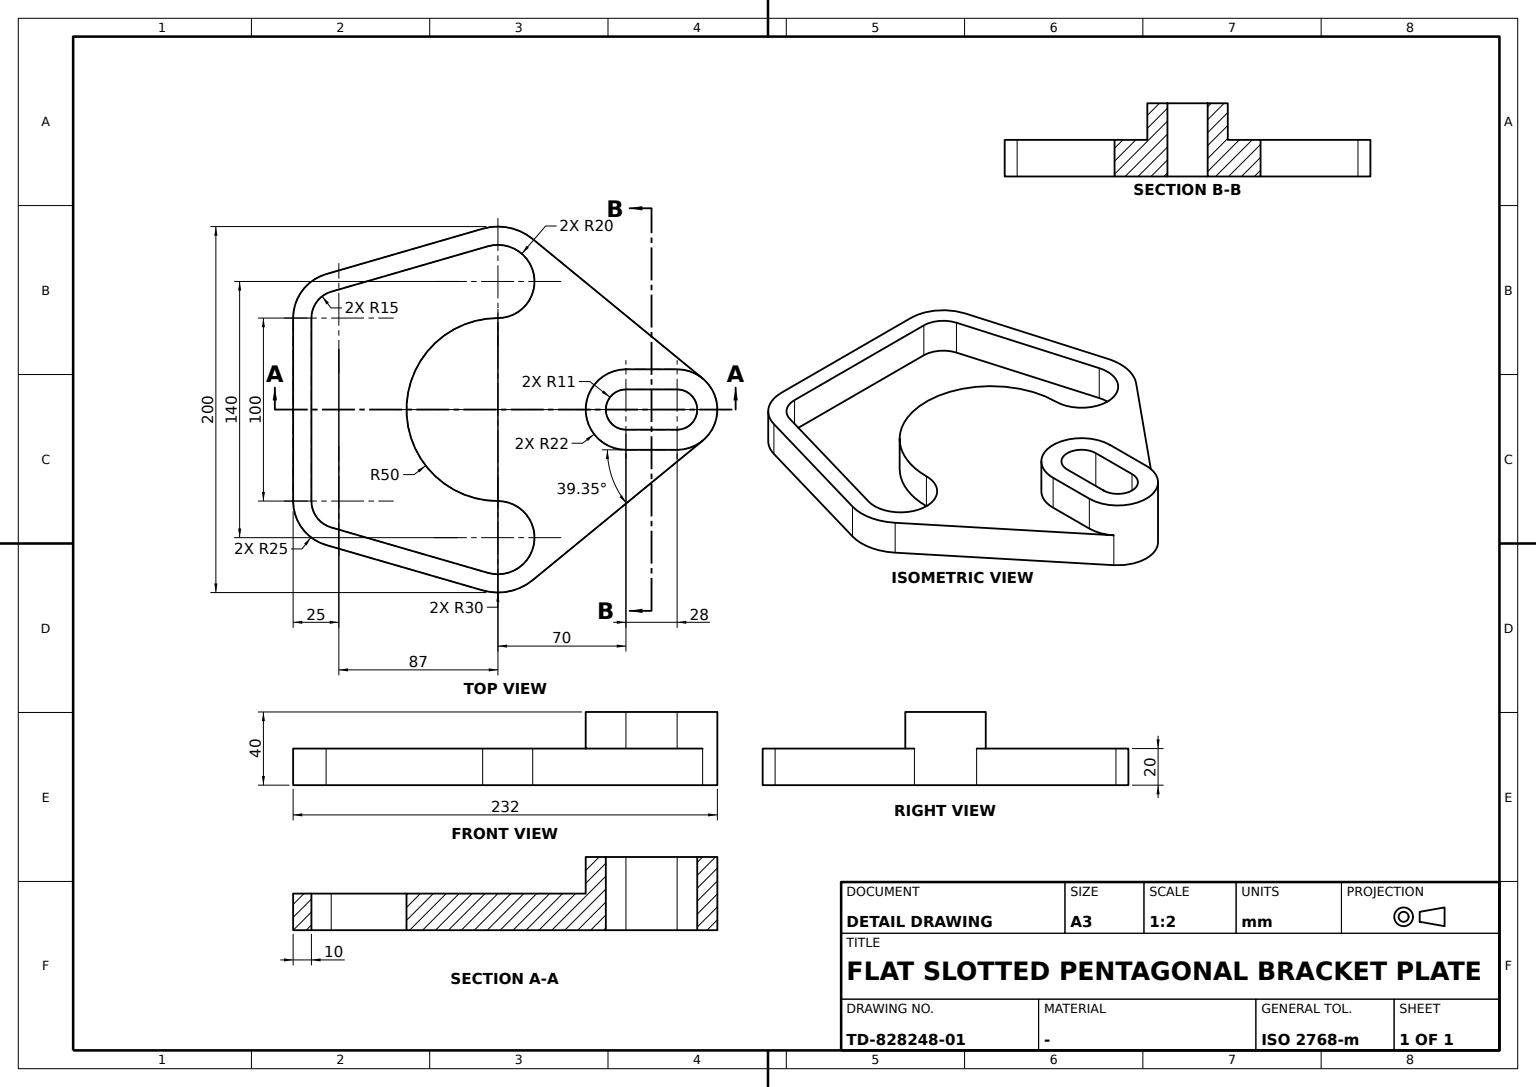
ISO-10303-21;
HEADER;
FILE_DESCRIPTION((''),'2;1');
FILE_NAME('','',(''),(''),'','','');
FILE_SCHEMA(('AUTOMOTIVE_DESIGN'));
ENDSEC;
DATA;
#1=APPLICATION_CONTEXT('');
#2=PRODUCT_CONTEXT('',#1,'mechanical');
#3=PRODUCT('','','',(#2));
#4=PRODUCT_DEFINITION_FORMATION('','',#3);
#5=PRODUCT_DEFINITION_CONTEXT('',#1,'design');
#6=PRODUCT_DEFINITION('','',#4,#5);
#7=PRODUCT_DEFINITION_SHAPE('','',#6);
#8=(LENGTH_UNIT()NAMED_UNIT(*)SI_UNIT(.MILLI.,.METRE.));
#9=(NAMED_UNIT(*)PLANE_ANGLE_UNIT()SI_UNIT($,.RADIAN.));
#10=(NAMED_UNIT(*)SI_UNIT($,.STERADIAN.)SOLID_ANGLE_UNIT());
#11=UNCERTAINTY_MEASURE_WITH_UNIT(LENGTH_MEASURE(0.005),#8,'distance_accuracy_value','');
#12=(GEOMETRIC_REPRESENTATION_CONTEXT(3)GLOBAL_UNCERTAINTY_ASSIGNED_CONTEXT((#11))GLOBAL_UNIT_ASSIGNED_CONTEXT((#8,#9,#10))REPRESENTATION_CONTEXT('',''));
#13=CARTESIAN_POINT('',(64.407517,-91.174142,0.));
#14=VERTEX_POINT('',#13);
#15=CARTESIAN_POINT('',(64.407517,-91.174142,-20.));
#16=VERTEX_POINT('',#15);
#17=CARTESIAN_POINT('',(64.407517,-91.174142,-10.));
#18=DIRECTION('',(0.,0.,1.));
#19=VECTOR('',#18,1000.);
#20=LINE('',#17,#19);
#21=EDGE_CURVE('',#14,#16,#20,.F.);
#22=ORIENTED_EDGE('',*,*,#21,.F.);
#23=CARTESIAN_POINT('',(89.210022,-5.565522,0.));
#24=VERTEX_POINT('',#23);
#25=DIRECTION('',(0.27827612,0.96050112,0.));
#26=VECTOR('',#25,1000.);
#27=LINE('',#13,#26);
#28=EDGE_CURVE('',#14,#24,#27,.T.);
#29=ORIENTED_EDGE('',*,*,#28,.T.);
#30=CARTESIAN_POINT('',(89.210022,-5.565522,-20.));
#31=VERTEX_POINT('',#30);
#32=CARTESIAN_POINT('',(89.210022,-5.565522,-10.));
#33=LINE('',#32,#19);
#34=EDGE_CURVE('',#24,#31,#33,.F.);
#35=ORIENTED_EDGE('',*,*,#34,.T.);
#36=LINE('',#15,#26);
#37=EDGE_CURVE('',#16,#31,#36,.T.);
#38=ORIENTED_EDGE('',*,*,#37,.F.);
#39=EDGE_LOOP('',(#22,#29,#35,#38));
#40=FACE_BOUND('',#39,.T.);
#41=DIRECTION('',(-0.96050112,0.27827612,0.));
#42=AXIS2_PLACEMENT_3D('',#13,#41,#25);
#43=PLANE('',#42);
#44=ADVANCED_FACE('',(#40),#43,.T.);
#45=CARTESIAN_POINT('',(-11.,70.,20.));
#46=VERTEX_POINT('',#45);
#47=CARTESIAN_POINT('',(-11.,70.,-20.));
#48=VERTEX_POINT('',#47);
#49=CARTESIAN_POINT('',(-11.,70.,10.));
#50=LINE('',#49,#19);
#51=EDGE_CURVE('',#46,#48,#50,.F.);
#52=ORIENTED_EDGE('',*,*,#51,.F.);
#53=CARTESIAN_POINT('',(11.,70.,20.));
#54=VERTEX_POINT('',#53);
#55=CARTESIAN_POINT('',(0.,70.,20.));
#56=DIRECTION('',(1.,0.,0.));
#57=AXIS2_PLACEMENT_3D('',#55,#18,#56);
#58=CIRCLE('',#57,11.);
#59=EDGE_CURVE('',#46,#54,#58,.T.);
#60=ORIENTED_EDGE('',*,*,#59,.T.);
#61=CARTESIAN_POINT('',(11.,70.,-20.));
#62=VERTEX_POINT('',#61);
#63=CARTESIAN_POINT('',(11.,70.,10.));
#64=LINE('',#63,#19);
#65=EDGE_CURVE('',#54,#62,#64,.F.);
#66=ORIENTED_EDGE('',*,*,#65,.T.);
#67=CARTESIAN_POINT('',(0.,70.,-20.));
#68=AXIS2_PLACEMENT_3D('',#67,#18,#56);
#69=CIRCLE('',#68,11.);
#70=EDGE_CURVE('',#48,#62,#69,.T.);
#71=ORIENTED_EDGE('',*,*,#70,.F.);
#72=EDGE_LOOP('',(#52,#60,#66,#71));
#73=FACE_BOUND('',#72,.T.);
#74=CARTESIAN_POINT('',(0.,70.,10.));
#75=AXIS2_PLACEMENT_3D('',#74,#18,#56);
#76=CYLINDRICAL_SURFACE('',#75,11.);
#77=ADVANCED_FACE('',(#73),#76,.F.);
#78=CARTESIAN_POINT('',(98.815034,-8.348284,-20.));
#79=VERTEX_POINT('',#78);
#80=CARTESIAN_POINT('',(93.199784,19.020254,-20.));
#81=VERTEX_POINT('',#80);
#82=CARTESIAN_POINT('',(70.,0.,-20.));
#83=AXIS2_PLACEMENT_3D('',#82,#18,#56);
#84=CIRCLE('',#83,30.);
#85=EDGE_CURVE('',#79,#81,#84,.T.);
#86=ORIENTED_EDGE('',*,*,#85,.T.);
#87=CARTESIAN_POINT('',(93.199784,19.020254,0.));
#88=VERTEX_POINT('',#87);
#89=CARTESIAN_POINT('',(93.199784,19.020254,-10.));
#90=LINE('',#89,#19);
#91=EDGE_CURVE('',#88,#81,#90,.F.);
#92=ORIENTED_EDGE('',*,*,#91,.F.);
#93=CARTESIAN_POINT('',(98.815034,-8.348284,0.));
#94=VERTEX_POINT('',#93);
#95=CARTESIAN_POINT('',(70.,0.,0.));
#96=AXIS2_PLACEMENT_3D('',#95,#18,#56);
#97=CIRCLE('',#96,30.);
#98=EDGE_CURVE('',#94,#88,#97,.T.);
#99=ORIENTED_EDGE('',*,*,#98,.F.);
#100=CARTESIAN_POINT('',(98.815034,-8.348284,-10.));
#101=LINE('',#100,#19);
#102=EDGE_CURVE('',#94,#79,#101,.F.);
#103=ORIENTED_EDGE('',*,*,#102,.T.);
#104=EDGE_LOOP('',(#86,#92,#99,#103));
#105=FACE_BOUND('',#104,.T.);
#106=CARTESIAN_POINT('',(70.,0.,-10.));
#107=AXIS2_PLACEMENT_3D('',#106,#18,#56);
#108=CYLINDRICAL_SURFACE('',#107,30.);
#109=ADVANCED_FACE('',(#105),#108,.T.);
#110=CARTESIAN_POINT('',(22.,70.,0.));
#111=VERTEX_POINT('',#110);
#112=CARTESIAN_POINT('',(22.,70.,20.));
#113=VERTEX_POINT('',#112);
#114=CARTESIAN_POINT('',(22.,70.,10.));
#115=LINE('',#114,#19);
#116=EDGE_CURVE('',#111,#113,#115,.T.);
#117=ORIENTED_EDGE('',*,*,#116,.T.);
#118=CARTESIAN_POINT('',(-22.,70.,20.));
#119=VERTEX_POINT('',#118);
#120=CIRCLE('',#57,22.);
#121=EDGE_CURVE('',#119,#113,#120,.T.);
#122=ORIENTED_EDGE('',*,*,#121,.F.);
#123=CARTESIAN_POINT('',(-22.,70.,0.));
#124=VERTEX_POINT('',#123);
#125=CARTESIAN_POINT('',(-22.,70.,10.));
#126=LINE('',#125,#19);
#127=EDGE_CURVE('',#124,#119,#126,.T.);
#128=ORIENTED_EDGE('',*,*,#127,.F.);
#129=CARTESIAN_POINT('',(0.,70.,0.));
#130=AXIS2_PLACEMENT_3D('',#129,#18,#56);
#131=CIRCLE('',#130,22.);
#132=EDGE_CURVE('',#124,#111,#131,.T.);
#133=ORIENTED_EDGE('',*,*,#132,.T.);
#134=EDGE_LOOP('',(#117,#122,#128,#133));
#135=FACE_BOUND('',#134,.T.);
#136=CYLINDRICAL_SURFACE('',#75,22.);
#137=ADVANCED_FACE('',(#135),#136,.T.);
#138=CARTESIAN_POINT('',(-64.407517,-91.174142,0.));
#139=VERTEX_POINT('',#138);
#140=CARTESIAN_POINT('',(-89.210022,-5.565522,0.));
#141=VERTEX_POINT('',#140);
#142=DIRECTION('',(-0.27827612,0.96050112,0.));
#143=VECTOR('',#142,1000.);
#144=LINE('',#138,#143);
#145=EDGE_CURVE('',#139,#141,#144,.T.);
#146=ORIENTED_EDGE('',*,*,#145,.F.);
#147=CARTESIAN_POINT('',(-64.407517,-91.174142,-20.));
#148=VERTEX_POINT('',#147);
#149=CARTESIAN_POINT('',(-64.407517,-91.174142,-10.));
#150=LINE('',#149,#19);
#151=EDGE_CURVE('',#139,#148,#150,.F.);
#152=ORIENTED_EDGE('',*,*,#151,.T.);
#153=CARTESIAN_POINT('',(-89.210022,-5.565522,-20.));
#154=VERTEX_POINT('',#153);
#155=LINE('',#147,#143);
#156=EDGE_CURVE('',#148,#154,#155,.T.);
#157=ORIENTED_EDGE('',*,*,#156,.T.);
#158=CARTESIAN_POINT('',(-89.210022,-5.565522,-10.));
#159=LINE('',#158,#19);
#160=EDGE_CURVE('',#141,#154,#159,.F.);
#161=ORIENTED_EDGE('',*,*,#160,.F.);
#162=EDGE_LOOP('',(#146,#152,#157,#161));
#163=FACE_BOUND('',#162,.T.);
#164=DIRECTION('',(-0.96050112,-0.27827612,0.));
#165=AXIS2_PLACEMENT_3D('',#138,#164,#142);
#166=PLANE('',#165);
#167=ADVANCED_FACE('',(#163),#166,.F.);
#168=CARTESIAN_POINT('',(11.,98.,20.));
#169=VERTEX_POINT('',#168);
#170=CARTESIAN_POINT('',(-11.,98.,20.));
#171=VERTEX_POINT('',#170);
#172=CARTESIAN_POINT('',(0.,98.,20.));
#173=AXIS2_PLACEMENT_3D('',#172,#18,#56);
#174=CIRCLE('',#173,11.);
#175=EDGE_CURVE('',#169,#171,#174,.T.);
#176=ORIENTED_EDGE('',*,*,#175,.T.);
#177=CARTESIAN_POINT('',(-11.,98.,-20.));
#178=VERTEX_POINT('',#177);
#179=CARTESIAN_POINT('',(-11.,98.,10.));
#180=LINE('',#179,#19);
#181=EDGE_CURVE('',#171,#178,#180,.F.);
#182=ORIENTED_EDGE('',*,*,#181,.T.);
#183=CARTESIAN_POINT('',(11.,98.,-20.));
#184=VERTEX_POINT('',#183);
#185=CARTESIAN_POINT('',(0.,98.,-20.));
#186=AXIS2_PLACEMENT_3D('',#185,#18,#56);
#187=CIRCLE('',#186,11.);
#188=EDGE_CURVE('',#184,#178,#187,.T.);
#189=ORIENTED_EDGE('',*,*,#188,.F.);
#190=CARTESIAN_POINT('',(11.,98.,10.));
#191=LINE('',#190,#19);
#192=EDGE_CURVE('',#169,#184,#191,.F.);
#193=ORIENTED_EDGE('',*,*,#192,.F.);
#194=EDGE_LOOP('',(#176,#182,#189,#193));
#195=FACE_BOUND('',#194,.T.);
#196=CARTESIAN_POINT('',(0.,98.,10.));
#197=AXIS2_PLACEMENT_3D('',#196,#18,#56);
#198=CYLINDRICAL_SURFACE('',#197,11.);
#199=ADVANCED_FACE('',(#195),#198,.F.);
#200=ORIENTED_EDGE('',*,*,#59,.F.);
#201=CARTESIAN_POINT('',(-11.,0.,20.));
#202=DIRECTION('',(0.,1.,0.));
#203=VECTOR('',#202,1000.);
#204=LINE('',#201,#203);
#205=EDGE_CURVE('',#46,#171,#204,.T.);
#206=ORIENTED_EDGE('',*,*,#205,.T.);
#207=ORIENTED_EDGE('',*,*,#175,.F.);
#208=CARTESIAN_POINT('',(11.,0.,20.));
#209=DIRECTION('',(0.,-1.,0.));
#210=VECTOR('',#209,1000.);
#211=LINE('',#208,#210);
#212=EDGE_CURVE('',#169,#54,#211,.T.);
#213=ORIENTED_EDGE('',*,*,#212,.T.);
#214=EDGE_LOOP('',(#200,#206,#207,#213));
#215=FACE_BOUND('',#214,.T.);
#216=CARTESIAN_POINT('',(22.,98.,20.));
#217=VERTEX_POINT('',#216);
#218=CARTESIAN_POINT('',(22.,0.,20.));
#219=LINE('',#218,#210);
#220=EDGE_CURVE('',#217,#113,#219,.T.);
#221=ORIENTED_EDGE('',*,*,#220,.F.);
#222=CARTESIAN_POINT('',(-22.,98.,20.));
#223=VERTEX_POINT('',#222);
#224=CIRCLE('',#173,22.);
#225=EDGE_CURVE('',#217,#223,#224,.T.);
#226=ORIENTED_EDGE('',*,*,#225,.T.);
#227=CARTESIAN_POINT('',(-22.,0.,20.));
#228=LINE('',#227,#203);
#229=EDGE_CURVE('',#119,#223,#228,.T.);
#230=ORIENTED_EDGE('',*,*,#229,.F.);
#231=ORIENTED_EDGE('',*,*,#121,.T.);
#232=EDGE_LOOP('',(#221,#226,#230,#231));
#233=FACE_BOUND('',#232,.T.);
#234=CARTESIAN_POINT('',(0.,0.,20.));
#235=AXIS2_PLACEMENT_3D('',#234,#18,#56);
#236=PLANE('',#235);
#237=ADVANCED_FACE('',(#215,#233),#236,.T.);
#238=CARTESIAN_POINT('',(-93.199784,19.020254,0.));
#239=VERTEX_POINT('',#238);
#240=CARTESIAN_POINT('',(-98.815034,-8.348284,0.));
#241=VERTEX_POINT('',#240);
#242=CARTESIAN_POINT('',(-70.,0.,0.));
#243=AXIS2_PLACEMENT_3D('',#242,#18,#56);
#244=CIRCLE('',#243,30.);
#245=EDGE_CURVE('',#239,#241,#244,.T.);
#246=ORIENTED_EDGE('',*,*,#245,.F.);
#247=CARTESIAN_POINT('',(-93.199784,19.020254,-20.));
#248=VERTEX_POINT('',#247);
#249=CARTESIAN_POINT('',(-93.199784,19.020254,-10.));
#250=LINE('',#249,#19);
#251=EDGE_CURVE('',#239,#248,#250,.F.);
#252=ORIENTED_EDGE('',*,*,#251,.T.);
#253=CARTESIAN_POINT('',(-98.815034,-8.348284,-20.));
#254=VERTEX_POINT('',#253);
#255=CARTESIAN_POINT('',(-70.,0.,-20.));
#256=AXIS2_PLACEMENT_3D('',#255,#18,#56);
#257=CIRCLE('',#256,30.);
#258=EDGE_CURVE('',#248,#254,#257,.T.);
#259=ORIENTED_EDGE('',*,*,#258,.T.);
#260=CARTESIAN_POINT('',(-98.815034,-8.348284,-10.));
#261=LINE('',#260,#19);
#262=EDGE_CURVE('',#241,#254,#261,.F.);
#263=ORIENTED_EDGE('',*,*,#262,.F.);
#264=EDGE_LOOP('',(#246,#252,#259,#263));
#265=FACE_BOUND('',#264,.T.);
#266=CARTESIAN_POINT('',(-70.,0.,-10.));
#267=AXIS2_PLACEMENT_3D('',#266,#18,#56);
#268=CYLINDRICAL_SURFACE('',#267,30.);
#269=ADVANCED_FACE('',(#265),#268,.T.);
#270=CARTESIAN_POINT('',(50.,0.,0.));
#271=VERTEX_POINT('',#270);
#272=CARTESIAN_POINT('',(50.,0.,-20.));
#273=VERTEX_POINT('',#272);
#274=CARTESIAN_POINT('',(50.,0.,-10.));
#275=LINE('',#274,#19);
#276=EDGE_CURVE('',#271,#273,#275,.F.);
#277=ORIENTED_EDGE('',*,*,#276,.F.);
#278=CARTESIAN_POINT('',(-50.,0.,0.));
#279=VERTEX_POINT('',#278);
#280=CARTESIAN_POINT('',(0.,0.,0.));
#281=AXIS2_PLACEMENT_3D('',#280,#18,#56);
#282=CIRCLE('',#281,50.);
#283=EDGE_CURVE('',#279,#271,#282,.T.);
#284=ORIENTED_EDGE('',*,*,#283,.F.);
#285=CARTESIAN_POINT('',(-50.,0.,-20.));
#286=VERTEX_POINT('',#285);
#287=CARTESIAN_POINT('',(-50.,0.,-10.));
#288=LINE('',#287,#19);
#289=EDGE_CURVE('',#279,#286,#288,.F.);
#290=ORIENTED_EDGE('',*,*,#289,.T.);
#291=CARTESIAN_POINT('',(0.,0.,-20.));
#292=AXIS2_PLACEMENT_3D('',#291,#18,#56);
#293=CIRCLE('',#292,50.);
#294=EDGE_CURVE('',#286,#273,#293,.T.);
#295=ORIENTED_EDGE('',*,*,#294,.T.);
#296=EDGE_LOOP('',(#277,#284,#290,#295));
#297=FACE_BOUND('',#296,.T.);
#298=CARTESIAN_POINT('',(0.,0.,-10.));
#299=AXIS2_PLACEMENT_3D('',#298,#18,#56);
#300=CYLINDRICAL_SURFACE('',#299,50.);
#301=ADVANCED_FACE('',(#297),#300,.T.);
#302=ORIENTED_EDGE('',*,*,#181,.F.);
#303=ORIENTED_EDGE('',*,*,#205,.F.);
#304=ORIENTED_EDGE('',*,*,#51,.T.);
#305=LINE('',#47,#210);
#306=EDGE_CURVE('',#178,#48,#305,.T.);
#307=ORIENTED_EDGE('',*,*,#306,.F.);
#308=EDGE_LOOP('',(#302,#303,#304,#307));
#309=FACE_BOUND('',#308,.T.);
#310=CARTESIAN_POINT('',(-11.,70.,0.));
#311=AXIS2_PLACEMENT_3D('',#310,#56,#202);
#312=PLANE('',#311);
#313=ADVANCED_FACE('',(#309),#312,.T.);
#314=ORIENTED_EDGE('',*,*,#65,.F.);
#315=ORIENTED_EDGE('',*,*,#212,.F.);
#316=ORIENTED_EDGE('',*,*,#192,.T.);
#317=LINE('',#183,#203);
#318=EDGE_CURVE('',#62,#184,#317,.T.);
#319=ORIENTED_EDGE('',*,*,#318,.F.);
#320=EDGE_LOOP('',(#314,#315,#316,#319));
#321=FACE_BOUND('',#320,.T.);
#322=CARTESIAN_POINT('',(11.,98.,0.));
#323=DIRECTION('',(-1.,0.,0.));
#324=AXIS2_PLACEMENT_3D('',#322,#323,#209);
#325=PLANE('',#324);
#326=ADVANCED_FACE('',(#321),#325,.T.);
#327=ORIENTED_EDGE('',*,*,#289,.F.);
#328=CIRCLE('',#243,20.);
#329=EDGE_CURVE('',#279,#141,#328,.T.);
#330=ORIENTED_EDGE('',*,*,#329,.T.);
#331=ORIENTED_EDGE('',*,*,#160,.T.);
#332=CIRCLE('',#256,20.);
#333=EDGE_CURVE('',#286,#154,#332,.T.);
#334=ORIENTED_EDGE('',*,*,#333,.F.);
#335=EDGE_LOOP('',(#327,#330,#331,#334));
#336=FACE_BOUND('',#335,.T.);
#337=CYLINDRICAL_SURFACE('',#267,20.);
#338=ADVANCED_FACE('',(#336),#337,.F.);
#339=CARTESIAN_POINT('',(-50.,-112.,0.));
#340=VERTEX_POINT('',#339);
#341=CARTESIAN_POINT('',(-50.,-112.,-20.));
#342=VERTEX_POINT('',#341);
#343=CARTESIAN_POINT('',(-50.,-112.,-10.));
#344=LINE('',#343,#19);
#345=EDGE_CURVE('',#340,#342,#344,.F.);
#346=ORIENTED_EDGE('',*,*,#345,.F.);
#347=CARTESIAN_POINT('',(-74.012528,-93.956903,0.));
#348=VERTEX_POINT('',#347);
#349=CARTESIAN_POINT('',(-50.,-87.,0.));
#350=AXIS2_PLACEMENT_3D('',#349,#18,#56);
#351=CIRCLE('',#350,25.);
#352=EDGE_CURVE('',#348,#340,#351,.T.);
#353=ORIENTED_EDGE('',*,*,#352,.F.);
#354=CARTESIAN_POINT('',(-74.012528,-93.956903,-20.));
#355=VERTEX_POINT('',#354);
#356=CARTESIAN_POINT('',(-74.012528,-93.956903,-10.));
#357=LINE('',#356,#19);
#358=EDGE_CURVE('',#348,#355,#357,.F.);
#359=ORIENTED_EDGE('',*,*,#358,.T.);
#360=CARTESIAN_POINT('',(-50.,-87.,-20.));
#361=AXIS2_PLACEMENT_3D('',#360,#18,#56);
#362=CIRCLE('',#361,25.);
#363=EDGE_CURVE('',#355,#342,#362,.T.);
#364=ORIENTED_EDGE('',*,*,#363,.T.);
#365=EDGE_LOOP('',(#346,#353,#359,#364));
#366=FACE_BOUND('',#365,.T.);
#367=CARTESIAN_POINT('',(-50.,-87.,-10.));
#368=AXIS2_PLACEMENT_3D('',#367,#18,#56);
#369=CYLINDRICAL_SURFACE('',#368,25.);
#370=ADVANCED_FACE('',(#366),#369,.T.);
#371=ORIENTED_EDGE('',*,*,#276,.T.);
#372=CIRCLE('',#83,20.);
#373=EDGE_CURVE('',#31,#273,#372,.T.);
#374=ORIENTED_EDGE('',*,*,#373,.F.);
#375=ORIENTED_EDGE('',*,*,#34,.F.);
#376=CIRCLE('',#96,20.);
#377=EDGE_CURVE('',#24,#271,#376,.T.);
#378=ORIENTED_EDGE('',*,*,#377,.T.);
#379=EDGE_LOOP('',(#371,#374,#375,#378));
#380=FACE_BOUND('',#379,.T.);
#381=CYLINDRICAL_SURFACE('',#107,20.);
#382=ADVANCED_FACE('',(#380),#381,.F.);
#383=ORIENTED_EDGE('',*,*,#116,.F.);
#384=CARTESIAN_POINT('',(22.,98.,0.));
#385=VERTEX_POINT('',#384);
#386=CARTESIAN_POINT('',(22.,0.,0.));
#387=LINE('',#386,#210);
#388=EDGE_CURVE('',#385,#111,#387,.T.);
#389=ORIENTED_EDGE('',*,*,#388,.F.);
#390=CARTESIAN_POINT('',(22.,98.,-10.));
#391=LINE('',#390,#19);
#392=EDGE_CURVE('',#385,#217,#391,.T.);
#393=ORIENTED_EDGE('',*,*,#392,.T.);
#394=ORIENTED_EDGE('',*,*,#220,.T.);
#395=EDGE_LOOP('',(#383,#389,#393,#394));
#396=FACE_BOUND('',#395,.T.);
#397=AXIS2_PLACEMENT_3D('',#384,#323,#209);
#398=PLANE('',#397);
#399=ADVANCED_FACE('',(#396),#398,.F.);
#400=CARTESIAN_POINT('',(-17.013175,111.948186,0.));
#401=VERTEX_POINT('',#400);
#402=CARTESIAN_POINT('',(-17.013175,111.948186,-20.));
#403=VERTEX_POINT('',#402);
#404=CARTESIAN_POINT('',(-17.013175,111.948186,-10.));
#405=LINE('',#404,#19);
#406=EDGE_CURVE('',#401,#403,#405,.F.);
#407=ORIENTED_EDGE('',*,*,#406,.F.);
#408=CARTESIAN_POINT('',(-22.,98.,0.));
#409=VERTEX_POINT('',#408);
#410=CARTESIAN_POINT('',(0.,98.,0.));
#411=AXIS2_PLACEMENT_3D('',#410,#18,#56);
#412=CIRCLE('',#411,22.);
#413=EDGE_CURVE('',#401,#409,#412,.T.);
#414=ORIENTED_EDGE('',*,*,#413,.T.);
#415=CARTESIAN_POINT('',(-22.,98.,-10.));
#416=LINE('',#415,#19);
#417=EDGE_CURVE('',#409,#223,#416,.T.);
#418=ORIENTED_EDGE('',*,*,#417,.T.);
#419=ORIENTED_EDGE('',*,*,#225,.F.);
#420=ORIENTED_EDGE('',*,*,#392,.F.);
#421=CARTESIAN_POINT('',(17.013175,111.948186,0.));
#422=VERTEX_POINT('',#421);
#423=EDGE_CURVE('',#385,#422,#412,.T.);
#424=ORIENTED_EDGE('',*,*,#423,.T.);
#425=CARTESIAN_POINT('',(17.013175,111.948186,-20.));
#426=VERTEX_POINT('',#425);
#427=CARTESIAN_POINT('',(17.013175,111.948186,-10.));
#428=LINE('',#427,#19);
#429=EDGE_CURVE('',#422,#426,#428,.F.);
#430=ORIENTED_EDGE('',*,*,#429,.T.);
#431=CIRCLE('',#186,22.);
#432=EDGE_CURVE('',#426,#403,#431,.T.);
#433=ORIENTED_EDGE('',*,*,#432,.T.);
#434=EDGE_LOOP('',(#407,#414,#418,#419,#420,#424,#430,#433));
#435=FACE_BOUND('',#434,.T.);
#436=CARTESIAN_POINT('',(0.,98.,-10.));
#437=AXIS2_PLACEMENT_3D('',#436,#18,#56);
#438=CYLINDRICAL_SURFACE('',#437,22.);
#439=ADVANCED_FACE('',(#435),#438,.T.);
#440=CARTESIAN_POINT('',(50.,-102.,-20.));
#441=VERTEX_POINT('',#440);
#442=CARTESIAN_POINT('',(50.,-87.,-20.));
#443=AXIS2_PLACEMENT_3D('',#442,#18,#56);
#444=CIRCLE('',#443,15.);
#445=EDGE_CURVE('',#441,#16,#444,.T.);
#446=ORIENTED_EDGE('',*,*,#445,.T.);
#447=ORIENTED_EDGE('',*,*,#37,.T.);
#448=ORIENTED_EDGE('',*,*,#373,.T.);
#449=ORIENTED_EDGE('',*,*,#294,.F.);
#450=ORIENTED_EDGE('',*,*,#333,.T.);
#451=ORIENTED_EDGE('',*,*,#156,.F.);
#452=CARTESIAN_POINT('',(-50.,-102.,-20.));
#453=VERTEX_POINT('',#452);
#454=CIRCLE('',#361,15.);
#455=EDGE_CURVE('',#148,#453,#454,.T.);
#456=ORIENTED_EDGE('',*,*,#455,.T.);
#457=VECTOR('',#323,1000.);
#458=LINE('',#440,#457);
#459=EDGE_CURVE('',#441,#453,#458,.T.);
#460=ORIENTED_EDGE('',*,*,#459,.F.);
#461=EDGE_LOOP('',(#446,#447,#448,#449,#450,#451,#456,#460));
#462=FACE_BOUND('',#461,.T.);
#463=CARTESIAN_POINT('',(74.012528,-93.956903,-20.));
#464=VERTEX_POINT('',#463);
#465=LINE('',#463,#26);
#466=EDGE_CURVE('',#464,#79,#465,.T.);
#467=ORIENTED_EDGE('',*,*,#466,.F.);
#468=CARTESIAN_POINT('',(50.,-112.,-20.));
#469=VERTEX_POINT('',#468);
#470=CIRCLE('',#443,25.);
#471=EDGE_CURVE('',#469,#464,#470,.T.);
#472=ORIENTED_EDGE('',*,*,#471,.F.);
#473=LINE('',#468,#457);
#474=EDGE_CURVE('',#469,#342,#473,.T.);
#475=ORIENTED_EDGE('',*,*,#474,.T.);
#476=ORIENTED_EDGE('',*,*,#363,.F.);
#477=LINE('',#354,#143);
#478=EDGE_CURVE('',#355,#254,#477,.T.);
#479=ORIENTED_EDGE('',*,*,#478,.T.);
#480=ORIENTED_EDGE('',*,*,#258,.F.);
#481=DIRECTION('',(-0.634008451,-0.773326117,0.));
#482=VECTOR('',#481,1000.);
#483=LINE('',#402,#482);
#484=EDGE_CURVE('',#403,#248,#483,.T.);
#485=ORIENTED_EDGE('',*,*,#484,.F.);
#486=ORIENTED_EDGE('',*,*,#432,.F.);
#487=DIRECTION('',(0.634008451,-0.773326117,0.));
#488=VECTOR('',#487,1000.);
#489=LINE('',#425,#488);
#490=EDGE_CURVE('',#426,#81,#489,.T.);
#491=ORIENTED_EDGE('',*,*,#490,.T.);
#492=ORIENTED_EDGE('',*,*,#85,.F.);
#493=EDGE_LOOP('',(#467,#472,#475,#476,#479,#480,#485,#486,#491,#492));
#494=FACE_BOUND('',#493,.T.);
#495=ORIENTED_EDGE('',*,*,#70,.T.);
#496=ORIENTED_EDGE('',*,*,#318,.T.);
#497=ORIENTED_EDGE('',*,*,#188,.T.);
#498=ORIENTED_EDGE('',*,*,#306,.T.);
#499=EDGE_LOOP('',(#495,#496,#497,#498));
#500=FACE_BOUND('',#499,.T.);
#501=PLANE('',#292);
#502=ADVANCED_FACE('',(#462,#494,#500),#501,.F.);
#503=ORIENTED_EDGE('',*,*,#466,.T.);
#504=ORIENTED_EDGE('',*,*,#102,.F.);
#505=CARTESIAN_POINT('',(74.012528,-93.956903,0.));
#506=VERTEX_POINT('',#505);
#507=LINE('',#505,#26);
#508=EDGE_CURVE('',#506,#94,#507,.T.);
#509=ORIENTED_EDGE('',*,*,#508,.F.);
#510=CARTESIAN_POINT('',(74.012528,-93.956903,-10.));
#511=LINE('',#510,#19);
#512=EDGE_CURVE('',#506,#464,#511,.F.);
#513=ORIENTED_EDGE('',*,*,#512,.T.);
#514=EDGE_LOOP('',(#503,#504,#509,#513));
#515=FACE_BOUND('',#514,.T.);
#516=AXIS2_PLACEMENT_3D('',#505,#41,#25);
#517=PLANE('',#516);
#518=ADVANCED_FACE('',(#515),#517,.F.);
#519=ORIENTED_EDGE('',*,*,#455,.F.);
#520=ORIENTED_EDGE('',*,*,#151,.F.);
#521=CARTESIAN_POINT('',(-50.,-102.,0.));
#522=VERTEX_POINT('',#521);
#523=CIRCLE('',#350,15.);
#524=EDGE_CURVE('',#139,#522,#523,.T.);
#525=ORIENTED_EDGE('',*,*,#524,.T.);
#526=CARTESIAN_POINT('',(-50.,-102.,-10.));
#527=LINE('',#526,#19);
#528=EDGE_CURVE('',#522,#453,#527,.F.);
#529=ORIENTED_EDGE('',*,*,#528,.T.);
#530=EDGE_LOOP('',(#519,#520,#525,#529));
#531=FACE_BOUND('',#530,.T.);
#532=CYLINDRICAL_SURFACE('',#368,15.);
#533=ADVANCED_FACE('',(#531),#532,.F.);
#534=ORIENTED_EDGE('',*,*,#429,.F.);
#535=LINE('',#421,#488);
#536=EDGE_CURVE('',#422,#88,#535,.T.);
#537=ORIENTED_EDGE('',*,*,#536,.T.);
#538=ORIENTED_EDGE('',*,*,#91,.T.);
#539=ORIENTED_EDGE('',*,*,#490,.F.);
#540=EDGE_LOOP('',(#534,#537,#538,#539));
#541=FACE_BOUND('',#540,.T.);
#542=DIRECTION('',(0.773326117,0.634008451,0.));
#543=AXIS2_PLACEMENT_3D('',#421,#542,#487);
#544=PLANE('',#543);
#545=ADVANCED_FACE('',(#541),#544,.T.);
#546=CARTESIAN_POINT('',(-22.,0.,0.));
#547=LINE('',#546,#203);
#548=EDGE_CURVE('',#124,#409,#547,.T.);
#549=ORIENTED_EDGE('',*,*,#548,.F.);
#550=ORIENTED_EDGE('',*,*,#127,.T.);
#551=ORIENTED_EDGE('',*,*,#229,.T.);
#552=ORIENTED_EDGE('',*,*,#417,.F.);
#553=EDGE_LOOP('',(#549,#550,#551,#552));
#554=FACE_BOUND('',#553,.T.);
#555=AXIS2_PLACEMENT_3D('',#123,#56,#202);
#556=PLANE('',#555);
#557=ADVANCED_FACE('',(#554),#556,.F.);
#558=CARTESIAN_POINT('',(50.,-102.,0.));
#559=VERTEX_POINT('',#558);
#560=CARTESIAN_POINT('',(50.,-102.,-10.));
#561=LINE('',#560,#19);
#562=EDGE_CURVE('',#559,#441,#561,.F.);
#563=ORIENTED_EDGE('',*,*,#562,.T.);
#564=ORIENTED_EDGE('',*,*,#459,.T.);
#565=ORIENTED_EDGE('',*,*,#528,.F.);
#566=LINE('',#558,#457);
#567=EDGE_CURVE('',#559,#522,#566,.T.);
#568=ORIENTED_EDGE('',*,*,#567,.F.);
#569=EDGE_LOOP('',(#563,#564,#565,#568));
#570=FACE_BOUND('',#569,.T.);
#571=AXIS2_PLACEMENT_3D('',#558,#209,#323);
#572=PLANE('',#571);
#573=ADVANCED_FACE('',(#570),#572,.F.);
#574=ORIENTED_EDGE('',*,*,#329,.F.);
#575=ORIENTED_EDGE('',*,*,#283,.T.);
#576=ORIENTED_EDGE('',*,*,#377,.F.);
#577=ORIENTED_EDGE('',*,*,#28,.F.);
#578=CARTESIAN_POINT('',(50.,-87.,0.));
#579=AXIS2_PLACEMENT_3D('',#578,#18,#56);
#580=CIRCLE('',#579,15.);
#581=EDGE_CURVE('',#559,#14,#580,.T.);
#582=ORIENTED_EDGE('',*,*,#581,.F.);
#583=ORIENTED_EDGE('',*,*,#567,.T.);
#584=ORIENTED_EDGE('',*,*,#524,.F.);
#585=ORIENTED_EDGE('',*,*,#145,.T.);
#586=EDGE_LOOP('',(#574,#575,#576,#577,#582,#583,#584,#585));
#587=FACE_BOUND('',#586,.T.);
#588=LINE('',#347,#143);
#589=EDGE_CURVE('',#348,#241,#588,.T.);
#590=ORIENTED_EDGE('',*,*,#589,.F.);
#591=ORIENTED_EDGE('',*,*,#352,.T.);
#592=CARTESIAN_POINT('',(50.,-112.,0.));
#593=VERTEX_POINT('',#592);
#594=LINE('',#592,#457);
#595=EDGE_CURVE('',#593,#340,#594,.T.);
#596=ORIENTED_EDGE('',*,*,#595,.F.);
#597=CIRCLE('',#579,25.);
#598=EDGE_CURVE('',#593,#506,#597,.T.);
#599=ORIENTED_EDGE('',*,*,#598,.T.);
#600=ORIENTED_EDGE('',*,*,#508,.T.);
#601=ORIENTED_EDGE('',*,*,#98,.T.);
#602=ORIENTED_EDGE('',*,*,#536,.F.);
#603=ORIENTED_EDGE('',*,*,#423,.F.);
#604=ORIENTED_EDGE('',*,*,#388,.T.);
#605=ORIENTED_EDGE('',*,*,#132,.F.);
#606=ORIENTED_EDGE('',*,*,#548,.T.);
#607=ORIENTED_EDGE('',*,*,#413,.F.);
#608=LINE('',#400,#482);
#609=EDGE_CURVE('',#401,#239,#608,.T.);
#610=ORIENTED_EDGE('',*,*,#609,.T.);
#611=ORIENTED_EDGE('',*,*,#245,.T.);
#612=EDGE_LOOP('',(#590,#591,#596,#599,#600,#601,#602,#603,#604,#605,#606,#607,#610,#611));
#613=FACE_BOUND('',#612,.T.);
#614=PLANE('',#281);
#615=ADVANCED_FACE('',(#587,#613),#614,.T.);
#616=ORIENTED_EDGE('',*,*,#445,.F.);
#617=ORIENTED_EDGE('',*,*,#562,.F.);
#618=ORIENTED_EDGE('',*,*,#581,.T.);
#619=ORIENTED_EDGE('',*,*,#21,.T.);
#620=EDGE_LOOP('',(#616,#617,#618,#619));
#621=FACE_BOUND('',#620,.T.);
#622=CARTESIAN_POINT('',(50.,-87.,-10.));
#623=AXIS2_PLACEMENT_3D('',#622,#18,#56);
#624=CYLINDRICAL_SURFACE('',#623,15.);
#625=ADVANCED_FACE('',(#621),#624,.F.);
#626=ORIENTED_EDGE('',*,*,#589,.T.);
#627=ORIENTED_EDGE('',*,*,#262,.T.);
#628=ORIENTED_EDGE('',*,*,#478,.F.);
#629=ORIENTED_EDGE('',*,*,#358,.F.);
#630=EDGE_LOOP('',(#626,#627,#628,#629));
#631=FACE_BOUND('',#630,.T.);
#632=AXIS2_PLACEMENT_3D('',#347,#164,#142);
#633=PLANE('',#632);
#634=ADVANCED_FACE('',(#631),#633,.T.);
#635=ORIENTED_EDGE('',*,*,#595,.T.);
#636=ORIENTED_EDGE('',*,*,#345,.T.);
#637=ORIENTED_EDGE('',*,*,#474,.F.);
#638=CARTESIAN_POINT('',(50.,-112.,-10.));
#639=LINE('',#638,#19);
#640=EDGE_CURVE('',#593,#469,#639,.F.);
#641=ORIENTED_EDGE('',*,*,#640,.F.);
#642=EDGE_LOOP('',(#635,#636,#637,#641));
#643=FACE_BOUND('',#642,.T.);
#644=AXIS2_PLACEMENT_3D('',#592,#209,#323);
#645=PLANE('',#644);
#646=ADVANCED_FACE('',(#643),#645,.T.);
#647=ORIENTED_EDGE('',*,*,#251,.F.);
#648=ORIENTED_EDGE('',*,*,#609,.F.);
#649=ORIENTED_EDGE('',*,*,#406,.T.);
#650=ORIENTED_EDGE('',*,*,#484,.T.);
#651=EDGE_LOOP('',(#647,#648,#649,#650));
#652=FACE_BOUND('',#651,.T.);
#653=DIRECTION('',(0.773326117,-0.634008451,0.));
#654=AXIS2_PLACEMENT_3D('',#400,#653,#481);
#655=PLANE('',#654);
#656=ADVANCED_FACE('',(#652),#655,.F.);
#657=ORIENTED_EDGE('',*,*,#512,.F.);
#658=ORIENTED_EDGE('',*,*,#598,.F.);
#659=ORIENTED_EDGE('',*,*,#640,.T.);
#660=ORIENTED_EDGE('',*,*,#471,.T.);
#661=EDGE_LOOP('',(#657,#658,#659,#660));
#662=FACE_BOUND('',#661,.T.);
#663=CYLINDRICAL_SURFACE('',#623,25.);
#664=ADVANCED_FACE('',(#662),#663,.T.);
#665=CLOSED_SHELL('',(#44,#77,#109,#137,#167,#199,#237,#269,#301,#313,#326,#338,#370,#382,#399,#439,#502,#518,#533,#545,#557,#573,#615,#625,#634,#646,#656,#664));
#666=MANIFOLD_SOLID_BREP('',#665);
#667=ADVANCED_BREP_SHAPE_REPRESENTATION('',(#666),#12);
#668=SHAPE_DEFINITION_REPRESENTATION(#7,#667);
ENDSEC;
END-ISO-10303-21;
